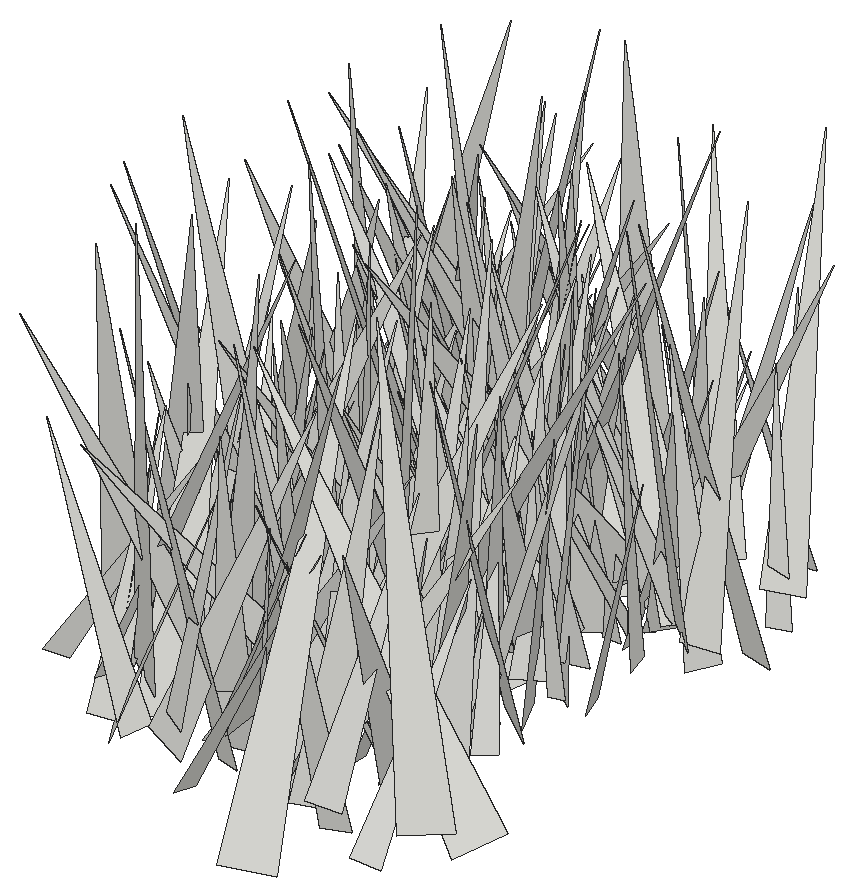
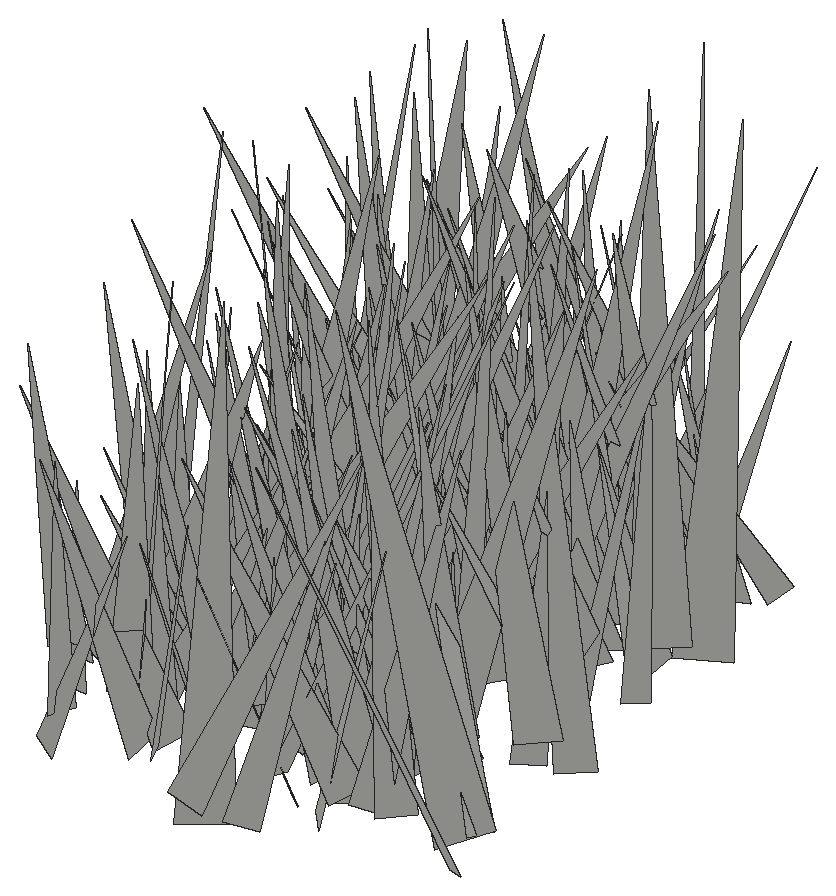
# SketchUp Ruby script. Lengths in inches.
U = 1.inch
M = Sketchup.active_model
def pt(a) = Geom::Point3d.new(a.map { |v| v * U })
def face(e, loops, mat)
  f = e.add_face(loops[0].map { |a| pt(a) })
  loops[1..].each { |l| e.add_face(l.map { |a| pt(a) }).erase! }
  f.material = f.back_material = mat if mat
  f
end
# faces: each face lists its corners as indices into pts; further lists are holes
def faces(e, pts, list, mat = nil) = list.each { |f| face(e, (f[0].is_a?(Array) ? f : [f]).map { |l| l.map { |i| pts[i] } }, mat) }
# xy, xz, yz: faces in a plane at the given z, y or x. An outline is a flat list of corners, or four numbers for a rectangle; further outlines are holes
def ring(l) = l.size == 4 ? [[l[0], l[1]], [l[2], l[1]], [l[2], l[3]], [l[0], l[3]]] : l.each_slice(2).to_a
def flat(e, list, mat, &to3) = list.each { |f| face(e, (f[0].is_a?(Array) ? f : [f]).map { |l| ring(l).map { |u, v| to3.(u, v) } }, mat) }
def xy(e, z, list, mat = nil) = flat(e, list, mat) { |x, y| [x, y, z] }
def xz(e, y, list, mat = nil) = flat(e, list, mat) { |x, z| [x, y, z] }
def yz(e, x, list, mat = nil) = flat(e, list, mat) { |y, z| [x, y, z] }
def lines(e, pts, list) = list.each { |a, b| e.add_line(pt(pts[a]), pt(pts[b])) }
# prism: a flat outline (further loops are holes) pulled along v
def prism(e, loops, v, mat = nil)
  f = face(e, loops, mat); d = Geom::Vector3d.new(v.map { |x| x * U })
  f.pushpull(f.normal.samedirection?(d) ? d.length : -d.length)
end
def box(e, o, s, mat = nil) = prism(e, [[o, [o[0] + s[0], o[1], o[2]], [o[0] + s[0], o[1] + s[1], o[2]], [o[0], o[1] + s[1], o[2]]]], [0, 0, s[2]], mat)
def at(x, y, z, deg = 0) = Geom::Transformation.translation(pt([x, y, z])) * Geom::Transformation.rotation(ORIGIN, Z_AXIS, deg.degrees)
def axes(o, x, y, z) = Geom::Transformation.new([*x, 0, *y, 0, *z, 0, *pt(o).to_a, 1])
def part(name) = M.definitions.add(name)
# library, detail: a bought-in or finely detailed component or shape, given as its bounding box
def library(name, o, s) = part(name).tap { |d| box(d.entities, o, s) }
def detail(e, o, s) = box(e.add_group.entities, o, s)
def put(e, d, t, mat = nil) = e.add_instance(d, t).tap { |i| i.material = mat if mat }
def group(e, t, mat = nil) = e.add_group.tap { |g| g.transformation = t; g.material = mat if mat }.entities
root = M.entities
c1 = part("fur_instance\#9")
p = [[0.8125,0,1.79],[0.67,-0.02,1.48],[0,-0.11,0],[0,0.11,0]]
faces(c1.entities,p,[[0,1,2,3]])
put(root,c1,axes([140.97,122.72,-28.22],[4.45979,0.0367,0.09292],[0.01604,-4.35825,0.95137],[-0.0986,0.95079,4.35729]))
put(root,c1,axes([143.02,123.39,-28.22],[2.46567,3.17158,1.58955],[3.37143,-2.69731,0.15219],[-1.10413,-1.15357,4.01439]))
put(root,c1,axes([145.18,120.2,-28.22],[-6.01479,5.28528,0.0687],[5.03484,5.76049,-2.36301],[1.60915,1.73181,7.65037]))
put(root,c1,axes([145.43,126.83,-28.22],[5.51839,-2.97407,0.09463],[-2.75984,-5.19025,-2.17974],[-1.11235,-1.87694,5.87762]))
put(root,c1,axes([141.22,123.61,-27.1],[3.86213,1.08614,0.2172],[1.09096,-3.86634,-0.0646],[-0.19154,-0.12107,4.01143]))
put(root,c1,axes([145.6875,123.53,-28.22],[0.77097,6.55392,2.92574],[6.60675,-1.79779,2.28627],[-2.8044,-2.43357,6.19042]))
put(root,c1,axes([145.86,122.76,-27.1],[-1.59343,4.55905,1.08338],[4.45907,1.82697,-1.12985],[1.44061,-0.61229,4.69546]))
put(root,c1,axes([141.12,125.19,-27.1],[7.51831,-0.309,0.51299],[-0.23256,-7.46002,-1.08516],[-0.55186,-1.06592,7.446]))
put(root,c1,axes([147.52,122.54,-28.22],[-1.08496,4.24211,0.2137],[4.12597,1.10497,-0.98676],[1.00871,0.04308,4.26602]))
put(root,c1,axes([137.42,125.39,-27.1],[-3.84702,-6.56229,2.86732],[-6.71624,4.43571,1.14075],[2.48541,1.82909,7.52076]))
put(root,c1,axes([149.05,123.33,-27.1],[2.27452,-5.56414,4.58515],[-6.58849,-3.55674,-1.04785],[-2.92831,3.68058,5.91904]))
put(root,c1,axes([137.87,124.46,-28.22],[-4.59292,1.38597,0.57425],[1.45174,4.5724,0.57548],[0.37836,-0.71958,4.76284]))
put(root,c1,axes([137.43,123.91,-28.22],[3.83341,2.26597,0.28943],[2.28132,-3.82668,-0.25597],[-0.11822,-0.36786,4.44568]))
put(root,c1,axes([141.03,124.56,-28.22],[-3.64938,-5.29226,1.74557],[-5.55344,3.28039,-1.66476],[-0.463,2.36729,6.20923]))
put(root,c1,axes([138.96,124.36,-28.22],[1.94999,6.06367,1.85826],[6.06829,-1.21894,-2.39034],[1.84311,-2.40204,5.90397]))
put(root,c1,axes([139.6,123.97,-27.1],[2.64561,4.33348,1.24236],[4.47199,-2.70465,-0.08904],[-0.56902,-1.10798,5.07645]))
put(root,c1,axes([144.87,126.34,-27.1],[-3.28468,-3.33783,0.1825],[-3.30088,3.27904,0.56182],[0.52783,-0.26523,4.64915]))
put(root,c1,axes([139.05,127.41,-28.22],[-7.29024,-1.74958,0.87658],[-1.40156,7.02793,2.37084],[1.36568,-2.12702,7.11251]))
put(root,c1,axes([144.41,124.19,-28.22],[-2.8521,5.31504,2.52319],[5.50682,3.39878,-0.93481],[2.07151,-1.71732,5.95905]))
put(root,c1,axes([149.37,125.29,-28.22],[-6.42815,4.45601,0.04956],[4.21627,6.0534,2.59983],[-1.44275,-2.16333,7.37686]))
put(root,c1,axes([139.79,126.31,-27.1],[3.06125,-3.87557,0.82155],[-3.90702,-3.12527,-0.1848],[-0.65588,0.52812,4.93529]))
put(root,c1,axes([140.46,128.47,-27.1],[-5.57045,-1.42182,0.3414],[-1.0257,4.7578,3.07884],[1.04215,-2.91715,4.85512]))
put(root,c1,axes([136.71,124.49,-28.22],[-1.136,4.49998,0.83575],[4.53043,1.22799,-0.4539],[0.65076,-0.69355,4.61891]))
put(root,c1,axes([140.26,125.35,-28.22],[4.87522,-3.55324,0.35007],[-3.38958,-4.41978,2.34354],[1.12198,2.08707,5.55888]))
put(root,c1,axes([135.28,127.69,-28.22],[4.47344,-6.57845,1.38646],[-6.62258,-4.59864,-0.45163],[-1.15746,0.88686,7.94253]))
put(root,c1,axes([143.74,125.67,-27.1],[-2.47,2.58512,1.49197],[2.74392,2.72878,-0.18549],[1.17462,-0.93843,3.57063]))
put(root,c1,axes([136.11,125.76,-28.22],[4.12014,1.91723,1.34742],[2.03951,-4.27599,-0.15214],[-1.154,-0.71202,4.54182]))
put(root,c1,axes([134.64,124.95,-27.1],[3.53802,-1.77872,0.68161],[-1.86523,-2.94336,2.00089],[0.38644,2.07817,3.41729]))
put(root,c1,axes([143.22,124.05,-28.22],[3.64416,1.65962,0.06909],[1.4569,-3.27351,1.789],[-0.79783,1.60274,3.58241]))
put(root,c1,axes([144.89,126.84,-28.22],[4.24569,0.44069,0.96407],[0.53821,-4.32495,-0.39327],[-0.91322,-0.50013,4.25034]))
put(root,c1,axes([141.4,127.53,-28.22],[1.75829,5.41715,3.42251],[6.36736,-1.87488,-0.30363],[-0.71818,-3.36006,5.68726]))
put(root,c1,axes([144.56,129.85,-27.1],[-0.28609,-7.90952,0.17476],[-7.91116,0.28452,-0.07401],[-0.06767,0.17732,7.91434]))
put(root,c1,axes([143.05,125.96,-28.22],[2.97178,5.39968,0.42783],[5.06638,-2.59832,-2.39825],[1.91609,-1.5044,5.67771]))
put(root,c1,axes([136.5,125,-27.1],[6.82155,0.82248,0.97272],[0.53436,-6.65794,1.88216],[-1.15634,1.77527,6.60814]))
put(root,c1,axes([142.84,124.55,-28.22],[1.53253,6.73152,0.42824],[6.72346,-1.5597,0.45586],[-0.5402,-0.31526,6.8887]))
put(root,c1,axes([144.89,129.125,-28.22],[7.23074,-0.77372,0.74856],[-0.57311,-7.06946,-1.77111],[-0.91134,-1.69312,7.05304]))
put(root,c1,axes([138.93,127.4,-27.1],[6.1687,-0.67373,2.21616],[-0.70194,-6.55164,-0.0379],[-2.20738,0.2006,6.20527]))
put(root,c1,axes([147.09,129.68,-27.1],[-3.51133,-6.12863,1.17286],[-5.90116,3.69891,1.66117],[2.0278,0.152,6.86513]))
put(root,c1,axes([135.39,129.46,-27.1],[5.72891,-5.77899,0.7373],[-5.79412,-5.75966,-0.12335],[-0.60698,0.43635,8.13646]))
put(root,c1,axes([136.48,125.95,-27.1],[3.1839,3.43631,0.24845],[3.39454,-3.18669,0.57383],[-0.5891,0.20968,4.64932]))
put(root,c1,axes([137.41,129.17,-27.1],[2.70621,-3.86796,1.26709],[-3.69816,-2.97221,-1.17466],[-1.70008,0.30833,4.57219]))
put(root,c1,axes([138.02,125.55,-28.22],[-5.32969,5.59283,1.04722],[5.46672,5.43108,-1.18331],[1.57839,0.07463,7.63447]))
put(root,c1,axes([144.82,128.36,-27.1],[-1.49682,6.02983,3.22428],[6.74332,1.8484,-0.32627],[1.1325,-3.03643,6.20426]))
put(root,c1,axes([142.8,126.23,-28.22],[-0.22471,7.89617,1.63504],[7.5306,0.79034,-2.78188],[2.88322,-1.44886,7.39332]))
put(root,c1,axes([145.1,128.71,-28.22],[1.79677,-5.19077,1.98742],[-5.55817,-1.66844,0.66734],[0.02536,2.09632,5.45226]))
put(root,c1,axes([137.97,128.72,-27.1],[3.87779,-2.1954,0.31482],[-2.2129,-3.78759,0.8446],[0.14815,0.88911,4.37535]))
put(root,c1,axes([141.53,128.34,-27.1],[-3.36679,-6.63148,1.92496],[-6.20382,1.96447,-4.08298],[-3.03226,3.34389,6.21619]))
put(root,c1,axes([146.7,126.95,-28.22],[-0.16365,8.04006,1.71484],[8.20749,0.06185,0.49328],[-0.46944,-1.72152,8.02659]))
put(root,c1,axes([143,129.53,-27.1],[-4.52397,-6.09316,3.51067],[-6.34353,5.33763,1.08955],[3.03497,2.07386,7.51038]))
put(root,c1,axes([144.96,128.37,-28.22],[-2.90723,2.3787,0.42473],[2.40963,2.90345,0.23285],[0.1797,-0.4498,3.74913]))
put(root,c1,axes([141.18,128.625,-28.22],[-3.40994,2.09099,1.78678],[2.1335,3.80705,-0.3836],[1.73581,-0.57158,3.98156]))
put(root,c1,axes([135.2,130.82,-28.22],[5.23051,-1.10724,0.78196],[-0.81536,-5.06,-1.7109],[-1.08287,-1.53819,5.06527]))
put(root,c1,axes([139.02,129.7,-27.1],[-7.80525,1.8691,2.4402],[2.24771,8.01322,1.05174],[2.09664,-1.63243,7.95672]))
put(root,c1,axes([139.97,129.23,-28.22],[-4.4516,-6.59475,1.62319],[-6.65602,3.85048,-2.61027],[-1.35017,2.76139,7.51625]))
put(root,c1,axes([147.49,127.86,-27.1],[-3.18847,2.06393,0.29466],[1.98964,3.17316,-0.69666],[0.62286,0.42918,3.73374]))
put(root,c1,axes([137.82,126.42,-27.1],[1.84381,6.83005,0.32521],[6.75707,-1.87158,0.99709],[-1.04756,-0.05069,7.00393]))
put(root,c1,axes([135.87,130.14,-27.1],[5.69454,1.71793,1.14191],[1.95584,-5.5622,-1.38552],[-0.6557,-1.67144,5.78441]))
put(root,c1,axes([145.58,130.52,-27.1],[5.69502,0.05498,1.49404],[0.36012,-5.7612,-1.16071],[-1.45103,-1.21405,5.57575]))
put(root,c1,axes([136,128.64,-28.22],[3.78689,-0.0231,1.24793],[-0.32688,-3.86581,0.92039],[-1.20458,0.97644,3.67342]))
put(root,c1,axes([146.01,127.82,-27.1],[2.63979,2.66437,0.28601],[2.37928,-2.51517,1.47039],[-1.23275,0.85099,3.4504]))
put(root,c1,axes([145.41,130.17,-28.22],[-6.59669,1.20746,2.1658],[1.44471,6.87425,0.5679],[2.0153,-0.97558,6.6822]))
put(root,c1,axes([144.15,129.46,-27.1],[3.92282,-1.4058,1.44453],[-1.66907,-4.03753,0.60333],[-1.1301,1.0833,4.1232]))
put(root,c1,axes([144.51,128.03,-28.22],[-0.26987,6.47949,0.83868],[6.52839,0.23411,0.29205],[-0.25936,-0.84936,6.47853]))
put(root,c1,axes([140.98,129.6,-28.22],[-7.32615,-2.19993,2.60741],[-2.57876,7.61493,-0.82074],[2.23345,1.57604,7.60517]))
put(root,c1,axes([139.31,134.0625,-27.1],[-5.60645,-3.595,0.79099],[-2.74257,5.04084,3.47133],[2.4552,-2.57833,5.68385]))
put(root,c1,axes([137.47,130.98,-27.1],[3.73633,3.15118,1.53756],[3.50493,-3.41917,-1.50964],[-0.09758,-2.15258,4.64878]))
put(root,c1,axes([140.33,131.6,-27.1],[-4.08347,2.98679,1.40676],[3.27171,3.36098,2.36101],[-0.44252,-2.71247,4.47451]))
put(root,c1,axes([136.8,131.86,-28.22],[-1.49518,-5.85947,1.8909],[-5.5495,2.12534,2.19783],[2.66683,1.13753,5.63369]))
put(root,c1,axes([136.1,132.41,-28.22],[-1.58112,-4.73276,0.31075],[-4.65779,1.61119,0.83937],[0.89473,0.02406,4.91878]))
put(root,c1,axes([143.7,126.99,-28.22],[7.42778,3.7642,0.92799],[3.25227,-7.14156,2.93652],[-2.11023,2.24305,7.79217]))
put(root,c1,axes([138.13,129.06,-28.22],[-3.1637,4.01487,0.30871],[3.99884,3.17867,-0.35895],[0.47305,-0.01931,5.09895]))
put(root,c1,axes([145.95,129.37,-27.1],[0.78964,4.34465,0.57519],[4.335,-0.86018,0.54605],[-0.64386,-0.46311,4.38193]))
put(root,c1,axes([145.29,132.81,-27.1],[4.67947,-2.49587,0.44393],[-2.29207,-4.56374,-1.49753],[-1.08298,-1.12554,5.08765]))
put(root,c1,axes([136.49,130.53,-27.1],[1.93796,6.92662,2.2466],[6.80944,-0.90011,-3.09877],[2.58009,-2.82714,6.49087]))
put(root,c1,axes([143.25,129.56,-27.1],[7.82793,-0.68601,0.13891],[-0.69946,-7.6099,1.83483],[0.02566,1.8399,7.64072]))
put(root,c1,axes([140.17,131.58,-27.1],[-3.26006,-5.04679,2.60885],[-5.29814,3.78652,0.70434],[2.05082,1.75965,5.96674]))
put(root,c1,axes([143.12,129.76,-28.22],[-2.96108,3.10315,0.36366],[3.04624,2.97875,-0.6142],[0.69442,0.16515,4.24503]))
put(root,c1,axes([146.5,128.64,-27.1],[4.01654,5.38759,0.39242],[5.219,-3.99648,1.45013],[-1.3936,0.56102,6.56169]))
put(root,c1,axes([144.28,132.83,-27.1],[-0.56318,-3.80765,0.20803],[-3.75255,0.51599,-0.71463],[-0.67806,0.30692,3.78215]))
put(root,c1,axes([145.8125,131.86,-28.22],[5.56182,2.46032,2.03104],[2.73268,-5.78042,-0.48104],[-1.64644,-1.28288,6.06264]))
put(root,c1,axes([143.14,133.34,-27.1],[-1.82356,-4.42835,0.39133],[-4.41286,1.85435,0.42054],[0.53859,0.19978,4.77062]))
put(root,c1,axes([141.38,132.9,-28.22],[-1.62801,-6.13851,1.48062],[-6.15059,1.19536,-1.80699],[-1.42958,1.84764,6.08822]))
put(root,c1,axes([146.3125,132.3125,-27.1],[-4.08433,-4.26667,3.28401],[-4.58243,4.91876,0.69141],[2.82675,1.80893,5.86585]))
put(root,c1,axes([147.05,131.59,-27.1],[0.66208,3.60921,1.19442],[3.54519,-1.02396,1.12897],[-1.37285,-0.90361,3.49144]))
put(root,c1,axes([143.88,130.32,-28.22],[-2.25135,6.36064,1.32657],[6.19225,2.52565,-1.60099],[1.96812,-0.67041,6.55463]))
put(root,c1,axes([143.62,134.21,-27.1],[0.2783,-5.0487,0.14304],[-4.93686,-0.24166,1.07529],[1.0664,0.19877,4.94071]))
put(root,c1,axes([140.7,130.7,-28.22],[-4.17558,2.72173,1.55923],[2.19552,4.39009,-1.78362],[2.24025,0.77057,4.65424]))
put(root,c1,axes([144.74,133.9375,-28.22],[1.51569,-5.39227,1.25729],[-5.41404,-1.71643,-0.83467],[-1.15995,0.96539,5.5387]))
put(root,c1,axes([136.17,131.34,-27.1],[-2.24412,3.20659,0.81725],[3.00578,2.38826,-1.11699],[1.38398,0.01256,3.75108]))
put(root,c1,axes([146.07,133.33,-27.1],[-0.62718,-6.98929,2.39617],[-7.29856,0.2117,-1.29283],[-1.15016,2.46782,6.89725]))
put(root,c1,axes([134.03,135.01,-28.22],[0.1957,-7.90399,1.09327],[-7.43409,0.21668,2.89722],[2.89871,1.0893,7.35646]))
put(root,c1,axes([145.1,133,-27.1],[-2.61332,3.50076,2.27341],[3.90248,3.00092,-0.13507],[1.48133,-1.72983,4.36652]))
put(root,c1,axes([144.62,133.52,-28.22],[-7.09229,4.18803,1.11711],[4.32642,6.70959,2.31334],[-0.26383,-2.55536,7.90497]))
put(root,c1,axes([142.74,133.07,-27.1],[-5.1387,-6.17044,1.38685],[-6.22365,4.61615,-2.52214],[-1.12419,2.64967,7.62361]))
put(root,c1,axes([141.57,135.15,-28.22],[-1.86711,-6.21996,0.83765],[-6.21183,1.95621,0.67975],[0.89595,0.60083,6.45848]))
put(root,c1,axes([146.86,133.39,-28.22],[3.94564,1.0984,0.79467],[1.2,-3.96752,-0.47419],[-0.63087,-0.67703,4.06813]))
put(root,c1,axes([141.08,135.26,-28.22],[1.40326,-4.201,0.43994],[-3.89786,-1.46649,-1.57071],[-1.62745,-0.10993,4.1413]))
put(root,c1,axes([135.36,135.48,-28.22],[4.86782,-2.47433,0.4659],[-2.27673,-4.75873,-1.48527],[-1.07512,-1.1257,5.25471]))
put(root,c1,axes([140.82,134.87,-27.1],[-1.81224,-5.34948,0.90018],[-5.42401,1.80193,-0.21131],[0.08596,0.92064,5.64415]))
put(root,c1,axes([139,132.5625,-27.1],[0.94432,5.62245,1.27282],[5.76049,-0.87093,-0.42662],[0.22085,-1.32412,5.68522]))
put(root,c1,axes([142.85,135.66,-27.1],[-6.28485,-0.79991,0.77187],[-0.56549,6.11624,1.73401],[0.95701,-1.63912,6.09364]))
put(root,c1,axes([144.49,137.89,-27.1],[4.16443,-6.48584,0.7003],[-5.50995,-3.94185,-3.74183],[-3.49241,-1.51483,6.7385]))
put(root,c1,axes([137.76,133.73,-27.1],[3.42061,-2.16163,2.16053],[-2.46149,-3.8706,0.02453],[-1.81151,1.17767,4.04631]))
put(root,c1,axes([145.9,133.3,-28.22],[3.38997,4.6985,2.258],[4.82742,-3.84601,0.75539],[-1.96736,-1.34115,5.74432]))
put(root,c1,axes([145.84,131.96,-27.1],[-5.09281,3.29268,0.78292],[3.01884,5.05892,-1.63872],[1.53013,0.9783,5.83893]))
put(root,c1,axes([145.91,136.14,-27.1],[-3.80651,-3.12707,0.03174],[-3.06593,3.74155,0.93273],[0.61617,-0.70095,4.83716]))
put(root,c1,axes([140.4,133.52,-27.1],[-1.29453,3.3269,0.92168],[3.25121,1.50588,-0.8692],[1.16077,-0.50757,3.46245]))
put(root,c1,axes([137.54,137.09,-28.22],[3.52912,-6.81057,1.30534],[-6.45742,-3.76145,-2.16695],[-2.52774,0.10047,7.35818]))
put(root,c1,axes([134.6875,135.875,-27.1],[2.49015,-6.48815,0.76577],[-6.33726,-2.19962,1.97082],[1.58797,1.39602,6.66429]))
put(root,c1,axes([147.6,134.48,-27.1],[-4.30965,-1.39305,1.63599],[-1.58025,4.5392,-0.29767],[1.45598,0.80324,4.51941]))
put(root,c1,axes([137.82,135.32,-27.1],[-7.27615,-1.41209,3.18772],[-1.2687,7.94356,0.62294],[3.24745,-0.06052,7.38568]))
put(root,c1,axes([147.51,136.55,-27.1],[-4.05006,-5.82532,2.03849],[-5.82326,4.4146,1.04584],[2.04438,1.03428,7.01738]))
put(root,c1,axes([135.39,134.2,-27.1],[4.11341,0.99659,0.14821],[0.94897,-4.04143,0.83763],[-0.33855,0.78037,4.1487]))
put(root,c1,axes([141.79,135.55,-28.22],[6.22111,3.48137,1.76986],[3.77865,-6.20685,-1.07301],[-0.98698,-1.81924,7.04775]))
put(root,c1,axes([140.625,132.6,-27.1],[5.39727,3.08007,0.18691],[2.81936,-5.07536,2.22356],[-1.25418,1.84558,5.80286]))
put(root,c1,axes([140.5625,135.34,-28.22],[4.00395,3.96639,1.91354],[4.25291,-4.1539,-0.28869],[-1.14309,-1.56151,5.62855]))
put(root,c1,axes([144.32,136.77,-28.22],[0.82361,-5.861,1.93807],[-5.93962,-1.28507,-1.3621],[-1.68178,1.66825,5.75972]))
put(root,c1,axes([143.02,137.78,-27.1],[-0.95701,-7.3765,1.52863],[-7.35851,1.24531,1.40248],[1.61303,1.30453,7.30491]))
put(root,c1,axes([144.125,137.6,-27.1],[-0.88156,-7.55851,1.51866],[-6.98391,0.13553,-3.37952],[-3.26533,1.75074,6.81814]))
put(root,c1,axes([139.36,136.22,-28.22],[-2.04031,-2.94511,1.87891],[-3.25881,2.38849,0.20512],[1.25863,1.41005,3.57693]))
put(root,c1,axes([139.82,138.75,-27.1],[0.11863,-7.1905,0.64579],[-7.08435,-0.24031,-1.37429],[-1.39009,0.61104,7.05894]))
put(root,c1,axes([139.85,138.46,-28.22],[6.98441,-2.34407,2.00985],[-1.86712,-7.16517,-1.86827],[-2.45928,-1.21733,7.12645]))
put(root,c1,axes([143.19,138.79,-28.22],[3.03189,-3.59681,0.02756],[-3.43565,-2.90654,-1.37057],[-1.06494,-0.8632,4.50011]))
put(root,c1,axes([147.14,137.05,-27.1],[-0.30638,-3.92044,1.36874],[-3.76361,-0.31774,-1.75256],[-1.75458,1.36615,3.52026]))
put(root,c1,axes([145.6875,138.04,-28.22],[3.85722,-2.97975,0.1804],[-2.96484,-3.85827,-0.33622],[-0.3481,-0.15623,4.86251]))
put(root,c1,axes([143.93,136.86,-28.22],[-4.50006,-1.01814,0.39176],[-1.03948,4.50642,-0.22865],[0.331,0.31016,4.60813]))
put(root,c1,axes([137.76,138.84,-28.22],[5.91516,-3.3432,1.65321],[-2.9566,-6.09276,-1.74243],[-2.27346,-0.77492,6.56735]))
put(root,c1,axes([144.9375,136.68,-28.22],[0.75971,3.71481,1.88794],[3.89435,-1.31575,1.02184],[-1.48263,-1.55251,3.65142]))
put(root,c1,axes([147.91,137.03,-28.22],[-4.24357,2.27798,1.78244],[2.54082,4.44811,0.36434],[1.38223,-1.18292,4.80254]))
put(root,c1,axes([141.78,138.32,-28.22],[6.97183,-3.45055,1.53762],[-3.37643,-7.13932,-0.71191],[-1.69419,0.0288,7.74635]))
put(root,c1,axes([141.375,138.78,-28.22],[-1.20375,-5.21342,0.24756],[-5.17288,1.15789,-0.76855],[-0.69453,0.4118,5.2951]))
put(root,c1,axes([145.65,137.79,-27.1],[-5.30182,-0.75056,0.88287],[-0.65483,5.35184,0.61739],[0.95603,-0.49663,5.31898]))
put(root,c1,axes([141.66,136.25,-27.1],[-7.85501,-1.13743,1.66782],[-1.3997,7.89692,-1.20666],[1.45472,1.45652,7.84468]))
put(root,c1,axes([139.68,135.51,-28.22],[5.78446,0.51407,0.77192],[0.25637,-5.57234,1.78981],[-0.89129,1.73346,5.52457]))
put(root,c1,axes([143.04,135.45,-27.1],[7.43701,2.08557,1.03262],[1.85087,-7.39668,1.60887],[-1.41074,1.29018,7.55449]))
put(root,c1,axes([142.72,135.79,-27.1],[-6.83852,1.49302,2.47832],[0.97247,7.17644,-1.63995],[2.72497,1.18576,6.80477]))
put(root,c1,axes([148.8,138.26,-28.22],[-2.90211,-6.23156,1.67253],[-6.44447,2.71044,-1.08359],[-0.31368,1.96803,6.78825]))
put(root,c1,axes([136.05,138,-28.22],[-0.14412,-3.47359,1.04669],[-3.58722,0.2928,0.47779],[0.54152,1.01518,3.44359]))
put(root,c1,axes([133.89,139.48,-28.22],[7.41722,0.99885,0.34739],[1.05742,-6.96886,-2.53978],[0.01548,-2.56338,7.04006]))
put(root,c1,axes([141.97,138.74,-27.1],[3.60736,-4.41491,0.21347],[-4.38405,-3.53869,0.89879],[0.56311,0.73233,5.62998]))
put(root,c1,axes([137.41,137.47,-28.22],[4.06898,-3.86093,0.67624],[-3.71406,-3.48612,2.44405],[1.25293,2.20473,5.04877]))
put(root,c1,axes([145.52,136.72,-28.22],[3.84083,1.33111,0.88578],[1.09907,-3.87194,1.0529],[-1.16125,0.73803,3.92622]))
put(root,c1,axes([135.52,137.87,-27.1],[0.91676,-3.52562,1.5814],[-3.59518,-0.18259,1.67709],[1.41617,1.81877,3.23385]))
put(root,c1,axes([148.35,136.32,-27.1],[-0.0106,6.43156,0.96228],[6.47441,-0.07994,0.60561],[-0.61077,-0.95901,6.403]))
put(root,c1,axes([138.625,137.67,-27.1],[-2.24155,-3.80564,2.54295],[-4.42537,2.52493,-0.12217],[1.16862,2.26183,4.41503]))
put(root,c1,axes([147.14,137.24,-27.1],[-3.95209,5.35159,0.47213],[5.26841,3.74586,1.6413],[-1.05182,-1.34553,6.44707]))
put(root,c1,axes([136.73,137.08,-27.1],[-2.92394,5.35838,1.35906],[5.44647,3.05552,-0.32925],[0.94614,-1.02969,6.09534]))
put(root,c1,axes([139.3,141.92,-27.1],[-7.53778,-2.79862,0.78068],[-2.32716,7.11502,3.03655],[1.73954,-2.60846,7.44512]))
put(root,c1,axes([138.09,139.72,-27.1],[-2.71876,-5.31687,1.33657],[-5.469,2.73415,-0.24823],[0.3815,1.3048,5.9665]))
put(root,c1,axes([138.12,136.65,-27.1],[-3.50119,3.09472,0.56001],[2.74674,3.41714,-1.71109],[1.53177,0.94611,4.34831]))
put(root,c1,axes([139.375,139.58,-28.22],[7.30646,0.41261,0.41525],[0.46932,-7.23653,-1.06747],[-0.34987,-1.09065,7.23983]))
put(root,c1,axes([145.6875,139.37,-28.22],[-0.35504,-4.51922,1.36303],[-4.31721,-0.2418,-1.92625],[-1.90863,1.3876,4.10353]))
put(root,c1,axes([145.49,137.97,-27.1],[0.85166,3.52496,0.51911],[3.494,-0.72175,-0.83136],[0.69768,-0.68839,3.5298]))
put(root,c1,axes([138.71,139.13,-27.1],[6.63487,-1.65212,1.91106],[-1.73662,-6.8834,0.0785],[-1.83462,0.54083,6.83702]))
put(root,c1,axes([139.9,139.02,-27.1],[-4.97089,0.8761,1.32855],[0.91857,5.13772,0.0489],[1.29955,-0.28038,5.04727]))
put(root,c1,axes([143.34,139.26,-28.22],[5.98361,0.11352,0.76596],[0.13466,-6.02993,-0.15823],[-0.76252,-0.17402,5.9826]))
put(root,c1,axes([139.88,138.25,-27.1],[-3.26703,2.9675,0.38966],[2.97957,3.27925,0.00816],[0.28293,-0.26806,4.41355]))
put(root,c1,axes([138,137.33,-28.22],[0.97806,5.36378,0.25201],[5.36787,-0.98334,0.09641],[-0.14015,-0.23057,5.45137]))
put(root,c1,axes([145.0625,140.13,-28.22],[4.53528,-3.04969,1.17101],[-3.07507,-4.66168,-0.23091],[-1.10265,0.45689,5.46041]))
put(root,c1,axes([135.15,141.71,-27.1],[6.92696,-1.79403,0.01467],[-1.72828,-6.68834,-1.86567],[-0.48147,-1.80253,6.90801]))
put(root,c1,axes([145.45,137.69,-28.22],[3.9731,1.20771,1.01378],[0.70264,-3.81635,1.79266],[-1.41159,1.49959,3.74573]))
put(root,c1,axes([139.75,138.07,-27.1],[0.8824,6.11345,1.2337],[6.18895,-1.01221,0.58924],[-0.77016,-1.12963,6.14863]))
put(root,c1,axes([135.98,141.96,-27.1],[1.38462,-5.25865,0.1546],[-5.22749,-1.39323,-0.57157],[-0.5921,0.00308,5.40776]))
put(root,c1,axes([143.68,138.85,-28.22],[-2.66965,3.73747,0.14274],[3.69986,2.61324,0.77338],[-0.54785,-0.56423,4.52743]))
put(root,c1,axes([143.55,139.76,-28.22],[-5.56985,2.38046,0.65327],[2.45077,5.52546,0.76123],[0.29505,-0.95874,6.00918]))
put(root,c1,axes([134.04,140,-28.22],[6.94828,-4.27135,1.74082],[-4.55894,-6.83788,1.41876],[-0.70067,2.13364,8.03182]))
put(root,c1,axes([145.42,140.4375,-27.1],[-5.46396,-3.21591,2.3792],[-3.43589,5.83542,-0.00311],[2.04873,1.20967,6.3401]))
put(root,c1,axes([138.6875,138.53,-28.22],[7.21368,2.51232,2.17903],[2.05011,-7.45745,1.81123],[-2.61859,1.08246,7.42081]))
put(root,c1,axes([148.17,140.06,-28.22],[-0.50007,3.75556,1.02909],[3.87876,0.38868,0.46638],[-0.34425,-1.07612,3.75989]))
put(root,c1,axes([144.61,139,-28.22],[1.96135,3.70682,0.36248],[3.45553,-1.96392,1.38604],[-1.38968,0.34826,3.95807]))
put(root,c1,axes([140.24,140.3125,-27.1],[-3.96056,0.86775,0.15545],[0.85071,3.94968,-0.37345],[0.23119,0.33194,4.03727]))
put(root,c1,axes([141.125,139.8,-27.1],[-3.9297,0.38452,0.60241],[0.18265,3.7953,-1.23109],[0.69093,1.18368,3.75164]))
put(root,c1,axes([137.38,140.49,-27.1],[4.47757,-3.00826,2.16701],[-3.51648,-4.52249,0.98776],[-1.1747,2.07164,5.30307]))
put(root,c1,axes([137.99,141.75,-28.22],[-3.38614,-3.10021,1.02366],[-3.22386,3.40798,-0.34286],[0.51569,0.94841,4.57818]))
put(root,c1,axes([144.02,141.59,-28.22],[-3.28529,-1.60429,1.12724],[-1.66632,3.44368,0.04462],[1.03333,0.45264,3.6558]))
put(root,c1,axes([144.06,140.68,-28.22],[5.41003,-2.25588,0.78895],[-2.38957,-5.13634,1.69936],[-0.03699,1.87321,5.60977]))
put(root,c1,axes([138.05,140.4375,-28.22],[-0.72846,5.64896,1.65026],[5.62241,1.15927,-1.48642],[1.73859,-1.38206,5.49837]))
put(root,c1,axes([136.96,141.64,-27.1],[4.24231,-3.44067,0.07958],[-3.18347,-3.87509,2.16585],[1.3077,1.72835,5.01442]))
put(root,c1,axes([145.77,140.51,-27.1],[-5.07407,3.61415,0.85454],[3.5922,5.14344,-0.42375],[0.94256,-0.14624,6.2152]))
put(root,c1,axes([133.07,141.67,-28.22],[4.19059,5.13354,0.34706],[4.85008,-3.79176,-2.47669],[1.71767,-1.81771,6.14657]))
put(root,c1,axes([148.21,140.16,-27.1],[-1.0825,6.58238,0.66021],[6.6005,1.02978,0.55528],[-0.44383,-0.73975,6.64764]))
put(root,c1,axes([139.28,141.19,-28.22],[2.54826,3.20038,0.28055],[3.20908,-2.5526,-0.02947],[-0.15164,-0.23787,4.09087]))
put(root,c1,axes([140.3,144.86,-27.1],[-0.06223,-5.95217,0.13196],[-5.73579,0.02457,-1.59678],[-1.59576,0.14382,5.73432]))
put(root,c1,axes([140.38,143.87,-28.22],[5.1556,-5.75467,2.21602],[-5.90961,-5.43588,-0.36737],[-1.76168,1.39363,7.71761]))
put(root,c1,axes([146.32,142.9,-27.1],[-3.33469,1.40616,1.82105],[1.56398,3.73727,-0.02186],[1.68745,-0.685,3.61897]))
put(root,c1,axes([138.22,144.89,-27.1],[2.83348,-4.00549,0.52306],[-3.76222,-2.8494,-1.43972],[-1.47079,-0.42795,4.69039]))
put(root,c1,axes([146.68,143.25,-28.22],[0.7235,3.49331,2.20248],[3.65755,-1.58024,1.30491],[-1.91742,-1.69623,3.32022]))
put(root,c1,axes([144.52,141.46,-28.22],[5.29795,0.17393,1.896],[-0.4687,-5.31448,1.7972],[-1.84537,1.84915,4.98684]))
